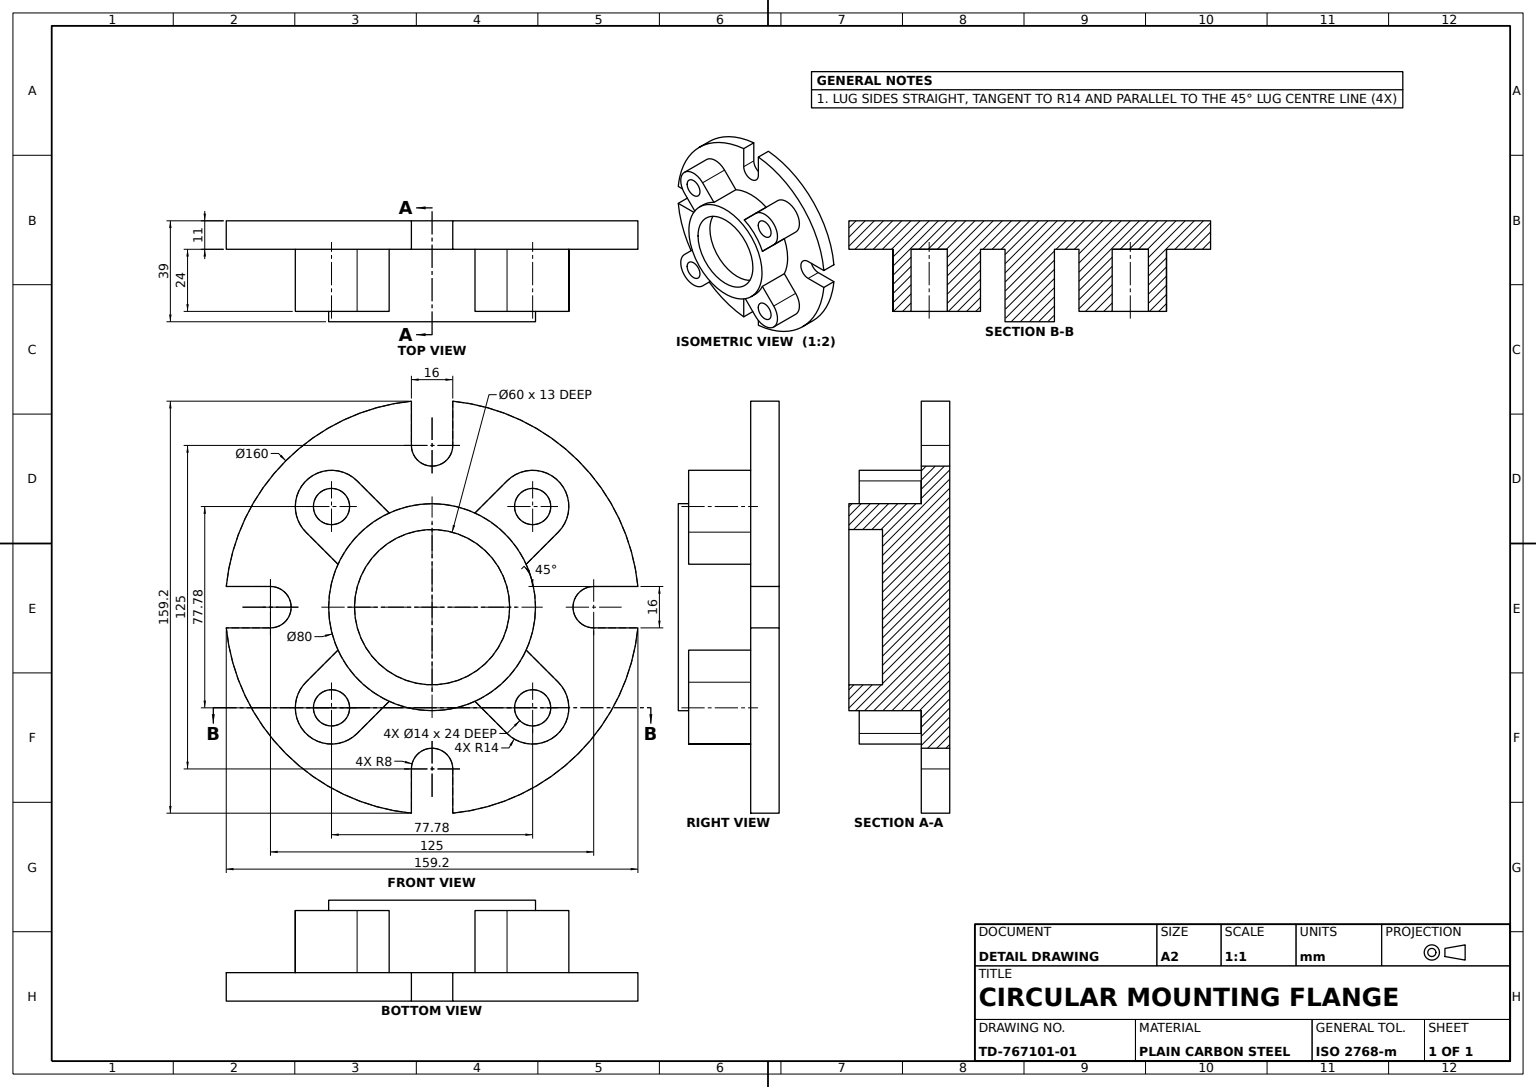
ISO-10303-21;
HEADER;
FILE_DESCRIPTION((''),'2;1');
FILE_NAME('','',(''),(''),'','','');
FILE_SCHEMA(('AUTOMOTIVE_DESIGN'));
ENDSEC;
DATA;
#1=APPLICATION_CONTEXT('');
#2=PRODUCT_CONTEXT('',#1,'mechanical');
#3=PRODUCT('','','',(#2));
#4=PRODUCT_DEFINITION_FORMATION('','',#3);
#5=PRODUCT_DEFINITION_CONTEXT('',#1,'design');
#6=PRODUCT_DEFINITION('','',#4,#5);
#7=PRODUCT_DEFINITION_SHAPE('','',#6);
#8=(LENGTH_UNIT()NAMED_UNIT(*)SI_UNIT(.MILLI.,.METRE.));
#9=(NAMED_UNIT(*)PLANE_ANGLE_UNIT()SI_UNIT($,.RADIAN.));
#10=(NAMED_UNIT(*)SI_UNIT($,.STERADIAN.)SOLID_ANGLE_UNIT());
#11=UNCERTAINTY_MEASURE_WITH_UNIT(LENGTH_MEASURE(1.E-05),#8,'distance_accuracy_value','');
#12=(GEOMETRIC_REPRESENTATION_CONTEXT(3)GLOBAL_UNCERTAINTY_ASSIGNED_CONTEXT((#11))GLOBAL_UNIT_ASSIGNED_CONTEXT((#8,#9,#10))REPRESENTATION_CONTEXT('',''));
#13=CARTESIAN_POINT('',(-79.598995,-8.,0.));
#14=VERTEX_POINT('',#13);
#15=CARTESIAN_POINT('',(-79.598995,-8.,11.));
#16=VERTEX_POINT('',#15);
#17=CARTESIAN_POINT('',(-79.598995,-8.,-13.));
#18=DIRECTION('',(0.,0.,1.));
#19=VECTOR('',#18,1000.);
#20=LINE('',#17,#19);
#21=EDGE_CURVE('',#14,#16,#20,.T.);
#22=ORIENTED_EDGE('',*,*,#21,.F.);
#23=CARTESIAN_POINT('',(-8.,-79.598995,0.));
#24=VERTEX_POINT('',#23);
#25=CARTESIAN_POINT('',(0.,0.,0.));
#26=DIRECTION('',(1.,0.,0.));
#27=AXIS2_PLACEMENT_3D('',#25,#18,#26);
#28=CIRCLE('',#27,80.);
#29=EDGE_CURVE('',#14,#24,#28,.T.);
#30=ORIENTED_EDGE('',*,*,#29,.T.);
#31=CARTESIAN_POINT('',(-8.,-79.598995,11.));
#32=VERTEX_POINT('',#31);
#33=CARTESIAN_POINT('',(-8.,-79.598995,-13.));
#34=LINE('',#33,#19);
#35=EDGE_CURVE('',#24,#32,#34,.T.);
#36=ORIENTED_EDGE('',*,*,#35,.T.);
#37=CARTESIAN_POINT('',(0.,0.,11.));
#38=AXIS2_PLACEMENT_3D('',#37,#18,#26);
#39=CIRCLE('',#38,80.);
#40=EDGE_CURVE('',#16,#32,#39,.T.);
#41=ORIENTED_EDGE('',*,*,#40,.F.);
#42=EDGE_LOOP('',(#22,#30,#36,#41));
#43=FACE_OUTER_BOUND('',#42,.T.);
#44=DIRECTION('',(0.,0.,-1.));
#45=DIRECTION('',(-1.,0.,0.));
#46=AXIS2_PLACEMENT_3D('',#37,#44,#45);
#47=CYLINDRICAL_SURFACE('',#46,80.);
#48=ADVANCED_FACE('',(#43),#47,.T.);
#49=CARTESIAN_POINT('',(-28.991378,-48.790368,35.));
#50=VERTEX_POINT('',#49);
#51=CARTESIAN_POINT('',(-16.595788,-36.394778,35.));
#52=VERTEX_POINT('',#51);
#53=DIRECTION('',(0.707106781,0.707106781,0.));
#54=VECTOR('',#53,1000.);
#55=LINE('',#51,#54);
#56=EDGE_CURVE('',#50,#52,#55,.T.);
#57=ORIENTED_EDGE('',*,*,#56,.F.);
#58=CARTESIAN_POINT('',(-28.991378,-48.790368,11.));
#59=VERTEX_POINT('',#58);
#60=VECTOR('',#44,1000.);
#61=LINE('',#49,#60);
#62=EDGE_CURVE('',#50,#59,#61,.T.);
#63=ORIENTED_EDGE('',*,*,#62,.T.);
#64=CARTESIAN_POINT('',(-16.595788,-36.394778,11.));
#65=VERTEX_POINT('',#64);
#66=LINE('',#64,#54);
#67=EDGE_CURVE('',#59,#65,#66,.T.);
#68=ORIENTED_EDGE('',*,*,#67,.T.);
#69=LINE('',#51,#60);
#70=EDGE_CURVE('',#52,#65,#69,.T.);
#71=ORIENTED_EDGE('',*,*,#70,.F.);
#72=EDGE_LOOP('',(#57,#63,#68,#71));
#73=FACE_OUTER_BOUND('',#72,.T.);
#74=DIRECTION('',(-0.707106781,0.707106781,0.));
#75=DIRECTION('',(-0.707106781,-0.707106781,0.));
#76=AXIS2_PLACEMENT_3D('',#51,#74,#75);
#77=PLANE('',#76);
#78=ADVANCED_FACE('',(#73),#77,.F.);
#79=CARTESIAN_POINT('',(45.890873,-38.890873,35.));
#80=VERTEX_POINT('',#79);
#81=CARTESIAN_POINT('',(31.890873,-38.890873,35.));
#82=VERTEX_POINT('',#81);
#83=CARTESIAN_POINT('',(38.890873,-38.890873,35.));
#84=DIRECTION('',(0.,-1.,0.));
#85=AXIS2_PLACEMENT_3D('',#83,#18,#84);
#86=CIRCLE('',#85,7.);
#87=EDGE_CURVE('',#80,#82,#86,.T.);
#88=ORIENTED_EDGE('',*,*,#87,.F.);
#89=EDGE_CURVE('',#82,#80,#86,.T.);
#90=ORIENTED_EDGE('',*,*,#89,.F.);
#91=EDGE_LOOP('',(#88,#90));
#92=FACE_BOUND('',#91,.T.);
#93=CARTESIAN_POINT('',(36.394778,-16.595788,35.));
#94=VERTEX_POINT('',#93);
#95=CARTESIAN_POINT('',(16.595788,-36.394778,35.));
#96=VERTEX_POINT('',#95);
#97=CARTESIAN_POINT('',(0.,0.,35.));
#98=AXIS2_PLACEMENT_3D('',#97,#44,#84);
#99=CIRCLE('',#98,40.);
#100=EDGE_CURVE('',#94,#96,#99,.T.);
#101=ORIENTED_EDGE('',*,*,#100,.T.);
#102=CARTESIAN_POINT('',(28.991378,-48.790368,35.));
#103=VERTEX_POINT('',#102);
#104=DIRECTION('',(0.707106781,-0.707106781,0.));
#105=VECTOR('',#104,1000.);
#106=LINE('',#95,#105);
#107=EDGE_CURVE('',#96,#103,#106,.T.);
#108=ORIENTED_EDGE('',*,*,#107,.T.);
#109=CARTESIAN_POINT('',(48.790368,-28.991378,35.));
#110=VERTEX_POINT('',#109);
#111=CIRCLE('',#85,14.);
#112=EDGE_CURVE('',#103,#110,#111,.T.);
#113=ORIENTED_EDGE('',*,*,#112,.T.);
#114=VECTOR('',#74,1000.);
#115=LINE('',#93,#114);
#116=EDGE_CURVE('',#110,#94,#115,.T.);
#117=ORIENTED_EDGE('',*,*,#116,.T.);
#118=EDGE_LOOP('',(#101,#108,#113,#117));
#119=FACE_OUTER_BOUND('',#118,.T.);
#120=AXIS2_PLACEMENT_3D('',#97,#18,#84);
#121=PLANE('',#120);
#122=ADVANCED_FACE('',(#92,#119),#121,.T.);
#123=CARTESIAN_POINT('',(62.5,8.,0.));
#124=VERTEX_POINT('',#123);
#125=CARTESIAN_POINT('',(62.5,8.,11.));
#126=VERTEX_POINT('',#125);
#127=CARTESIAN_POINT('',(62.5,8.,-13.));
#128=LINE('',#127,#19);
#129=EDGE_CURVE('',#124,#126,#128,.T.);
#130=ORIENTED_EDGE('',*,*,#129,.T.);
#131=CARTESIAN_POINT('',(62.5,-8.,11.));
#132=VERTEX_POINT('',#131);
#133=CARTESIAN_POINT('',(62.5,0.,11.));
#134=AXIS2_PLACEMENT_3D('',#133,#18,#26);
#135=CIRCLE('',#134,8.);
#136=EDGE_CURVE('',#126,#132,#135,.T.);
#137=ORIENTED_EDGE('',*,*,#136,.T.);
#138=CARTESIAN_POINT('',(62.5,-8.,0.));
#139=VERTEX_POINT('',#138);
#140=CARTESIAN_POINT('',(62.5,-8.,-13.));
#141=LINE('',#140,#19);
#142=EDGE_CURVE('',#139,#132,#141,.T.);
#143=ORIENTED_EDGE('',*,*,#142,.F.);
#144=CARTESIAN_POINT('',(62.5,0.,0.));
#145=AXIS2_PLACEMENT_3D('',#144,#18,#26);
#146=CIRCLE('',#145,8.);
#147=EDGE_CURVE('',#124,#139,#146,.T.);
#148=ORIENTED_EDGE('',*,*,#147,.F.);
#149=EDGE_LOOP('',(#130,#137,#143,#148));
#150=FACE_OUTER_BOUND('',#149,.T.);
#151=CARTESIAN_POINT('',(62.5,0.,-13.));
#152=AXIS2_PLACEMENT_3D('',#151,#18,#26);
#153=CYLINDRICAL_SURFACE('',#152,8.);
#154=ADVANCED_FACE('',(#150),#153,.F.);
#155=CARTESIAN_POINT('',(16.595788,36.394778,35.));
#156=VERTEX_POINT('',#155);
#157=CARTESIAN_POINT('',(36.394778,16.595788,35.));
#158=VERTEX_POINT('',#157);
#159=AXIS2_PLACEMENT_3D('',#97,#44,#26);
#160=CIRCLE('',#159,40.);
#161=EDGE_CURVE('',#156,#158,#160,.T.);
#162=ORIENTED_EDGE('',*,*,#161,.T.);
#163=CARTESIAN_POINT('',(48.790368,28.991378,35.));
#164=VERTEX_POINT('',#163);
#165=LINE('',#157,#54);
#166=EDGE_CURVE('',#158,#164,#165,.T.);
#167=ORIENTED_EDGE('',*,*,#166,.T.);
#168=CARTESIAN_POINT('',(28.991378,48.790368,35.));
#169=VERTEX_POINT('',#168);
#170=CARTESIAN_POINT('',(38.890873,38.890873,35.));
#171=AXIS2_PLACEMENT_3D('',#170,#18,#26);
#172=CIRCLE('',#171,14.);
#173=EDGE_CURVE('',#164,#169,#172,.T.);
#174=ORIENTED_EDGE('',*,*,#173,.T.);
#175=VECTOR('',#75,1000.);
#176=LINE('',#155,#175);
#177=EDGE_CURVE('',#169,#156,#176,.T.);
#178=ORIENTED_EDGE('',*,*,#177,.T.);
#179=EDGE_LOOP('',(#162,#167,#174,#178));
#180=FACE_OUTER_BOUND('',#179,.T.);
#181=CARTESIAN_POINT('',(31.890873,38.890873,35.));
#182=VERTEX_POINT('',#181);
#183=CARTESIAN_POINT('',(45.890873,38.890873,35.));
#184=VERTEX_POINT('',#183);
#185=CIRCLE('',#171,7.);
#186=EDGE_CURVE('',#182,#184,#185,.T.);
#187=ORIENTED_EDGE('',*,*,#186,.F.);
#188=EDGE_CURVE('',#184,#182,#185,.T.);
#189=ORIENTED_EDGE('',*,*,#188,.F.);
#190=EDGE_LOOP('',(#187,#189));
#191=FACE_BOUND('',#190,.T.);
#192=AXIS2_PLACEMENT_3D('',#97,#18,#26);
#193=PLANE('',#192);
#194=ADVANCED_FACE('',(#180,#191),#193,.T.);
#195=ORIENTED_EDGE('',*,*,#166,.F.);
#196=CARTESIAN_POINT('',(36.394778,16.595788,11.));
#197=VERTEX_POINT('',#196);
#198=LINE('',#157,#60);
#199=EDGE_CURVE('',#158,#197,#198,.T.);
#200=ORIENTED_EDGE('',*,*,#199,.T.);
#201=CARTESIAN_POINT('',(48.790368,28.991378,11.));
#202=VERTEX_POINT('',#201);
#203=LINE('',#196,#54);
#204=EDGE_CURVE('',#197,#202,#203,.T.);
#205=ORIENTED_EDGE('',*,*,#204,.T.);
#206=LINE('',#163,#60);
#207=EDGE_CURVE('',#164,#202,#206,.T.);
#208=ORIENTED_EDGE('',*,*,#207,.F.);
#209=EDGE_LOOP('',(#195,#200,#205,#208));
#210=FACE_OUTER_BOUND('',#209,.T.);
#211=AXIS2_PLACEMENT_3D('',#157,#74,#75);
#212=PLANE('',#211);
#213=ADVANCED_FACE('',(#210),#212,.F.);
#214=CARTESIAN_POINT('',(31.890873,-38.890873,11.));
#215=VERTEX_POINT('',#214);
#216=CARTESIAN_POINT('',(45.890873,-38.890873,11.));
#217=VERTEX_POINT('',#216);
#218=CARTESIAN_POINT('',(38.890873,-38.890873,11.));
#219=AXIS2_PLACEMENT_3D('',#218,#44,#26);
#220=CIRCLE('',#219,7.);
#221=EDGE_CURVE('',#215,#217,#220,.T.);
#222=ORIENTED_EDGE('',*,*,#221,.F.);
#223=EDGE_CURVE('',#217,#215,#220,.T.);
#224=ORIENTED_EDGE('',*,*,#223,.F.);
#225=EDGE_LOOP('',(#222,#224));
#226=FACE_OUTER_BOUND('',#225,.T.);
#227=PLANE('',#38);
#228=ADVANCED_FACE('',(#226),#227,.T.);
#229=CARTESIAN_POINT('',(8.,-79.598995,11.));
#230=VERTEX_POINT('',#229);
#231=CARTESIAN_POINT('',(79.598995,-8.,11.));
#232=VERTEX_POINT('',#231);
#233=EDGE_CURVE('',#230,#232,#39,.T.);
#234=ORIENTED_EDGE('',*,*,#233,.F.);
#235=CARTESIAN_POINT('',(8.,-79.598995,0.));
#236=VERTEX_POINT('',#235);
#237=CARTESIAN_POINT('',(8.,-79.598995,-13.));
#238=LINE('',#237,#19);
#239=EDGE_CURVE('',#236,#230,#238,.T.);
#240=ORIENTED_EDGE('',*,*,#239,.F.);
#241=CARTESIAN_POINT('',(79.598995,-8.,0.));
#242=VERTEX_POINT('',#241);
#243=EDGE_CURVE('',#236,#242,#28,.T.);
#244=ORIENTED_EDGE('',*,*,#243,.T.);
#245=CARTESIAN_POINT('',(79.598995,-8.,-13.));
#246=LINE('',#245,#19);
#247=EDGE_CURVE('',#242,#232,#246,.T.);
#248=ORIENTED_EDGE('',*,*,#247,.T.);
#249=EDGE_LOOP('',(#234,#240,#244,#248));
#250=FACE_OUTER_BOUND('',#249,.T.);
#251=ADVANCED_FACE('',(#250),#47,.T.);
#252=CARTESIAN_POINT('',(-45.890873,-38.890873,35.));
#253=VERTEX_POINT('',#252);
#254=CARTESIAN_POINT('',(-45.890873,-38.890873,11.));
#255=VERTEX_POINT('',#254);
#256=LINE('',#252,#60);
#257=EDGE_CURVE('',#253,#255,#256,.T.);
#258=ORIENTED_EDGE('',*,*,#257,.T.);
#259=CARTESIAN_POINT('',(-31.890873,-38.890873,11.));
#260=VERTEX_POINT('',#259);
#261=CARTESIAN_POINT('',(-38.890873,-38.890873,11.));
#262=AXIS2_PLACEMENT_3D('',#261,#44,#26);
#263=CIRCLE('',#262,7.);
#264=EDGE_CURVE('',#255,#260,#263,.T.);
#265=ORIENTED_EDGE('',*,*,#264,.T.);
#266=CARTESIAN_POINT('',(-31.890873,-38.890873,35.));
#267=VERTEX_POINT('',#266);
#268=LINE('',#266,#60);
#269=EDGE_CURVE('',#267,#260,#268,.T.);
#270=ORIENTED_EDGE('',*,*,#269,.F.);
#271=CARTESIAN_POINT('',(-38.890873,-38.890873,35.));
#272=AXIS2_PLACEMENT_3D('',#271,#18,#45);
#273=CIRCLE('',#272,7.);
#274=EDGE_CURVE('',#267,#253,#273,.T.);
#275=ORIENTED_EDGE('',*,*,#274,.T.);
#276=EDGE_LOOP('',(#258,#265,#270,#275));
#277=FACE_OUTER_BOUND('',#276,.T.);
#278=AXIS2_PLACEMENT_3D('',#271,#44,#45);
#279=CYLINDRICAL_SURFACE('',#278,7.);
#280=ADVANCED_FACE('',(#277),#279,.F.);
#281=CARTESIAN_POINT('',(-45.890873,38.890873,11.));
#282=VERTEX_POINT('',#281);
#283=CARTESIAN_POINT('',(-31.890873,38.890873,11.));
#284=VERTEX_POINT('',#283);
#285=CARTESIAN_POINT('',(-38.890873,38.890873,11.));
#286=AXIS2_PLACEMENT_3D('',#285,#44,#26);
#287=CIRCLE('',#286,7.);
#288=EDGE_CURVE('',#282,#284,#287,.T.);
#289=ORIENTED_EDGE('',*,*,#288,.T.);
#290=CARTESIAN_POINT('',(-31.890873,38.890873,35.));
#291=VERTEX_POINT('',#290);
#292=LINE('',#290,#60);
#293=EDGE_CURVE('',#291,#284,#292,.T.);
#294=ORIENTED_EDGE('',*,*,#293,.F.);
#295=CARTESIAN_POINT('',(-45.890873,38.890873,35.));
#296=VERTEX_POINT('',#295);
#297=CARTESIAN_POINT('',(-38.890873,38.890873,35.));
#298=DIRECTION('',(0.,1.,0.));
#299=AXIS2_PLACEMENT_3D('',#297,#18,#298);
#300=CIRCLE('',#299,7.);
#301=EDGE_CURVE('',#291,#296,#300,.T.);
#302=ORIENTED_EDGE('',*,*,#301,.T.);
#303=LINE('',#295,#60);
#304=EDGE_CURVE('',#296,#282,#303,.T.);
#305=ORIENTED_EDGE('',*,*,#304,.T.);
#306=EDGE_LOOP('',(#289,#294,#302,#305));
#307=FACE_OUTER_BOUND('',#306,.T.);
#308=AXIS2_PLACEMENT_3D('',#297,#44,#45);
#309=CYLINDRICAL_SURFACE('',#308,7.);
#310=ADVANCED_FACE('',(#307),#309,.F.);
#311=ORIENTED_EDGE('',*,*,#87,.T.);
#312=LINE('',#81,#60);
#313=EDGE_CURVE('',#82,#215,#312,.T.);
#314=ORIENTED_EDGE('',*,*,#313,.T.);
#315=ORIENTED_EDGE('',*,*,#221,.T.);
#316=LINE('',#79,#60);
#317=EDGE_CURVE('',#80,#217,#316,.T.);
#318=ORIENTED_EDGE('',*,*,#317,.F.);
#319=EDGE_LOOP('',(#311,#314,#315,#318));
#320=FACE_OUTER_BOUND('',#319,.T.);
#321=AXIS2_PLACEMENT_3D('',#83,#44,#45);
#322=CYLINDRICAL_SURFACE('',#321,7.);
#323=ADVANCED_FACE('',(#320),#322,.F.);
#324=CARTESIAN_POINT('',(-28.991378,48.790368,35.));
#325=VERTEX_POINT('',#324);
#326=CARTESIAN_POINT('',(-52.890873,38.890873,35.));
#327=VERTEX_POINT('',#326);
#328=CIRCLE('',#299,14.);
#329=EDGE_CURVE('',#325,#327,#328,.T.);
#330=ORIENTED_EDGE('',*,*,#329,.F.);
#331=CARTESIAN_POINT('',(-28.991378,48.790368,11.));
#332=VERTEX_POINT('',#331);
#333=LINE('',#324,#60);
#334=EDGE_CURVE('',#325,#332,#333,.T.);
#335=ORIENTED_EDGE('',*,*,#334,.T.);
#336=CARTESIAN_POINT('',(-52.890873,38.890873,11.));
#337=VERTEX_POINT('',#336);
#338=AXIS2_PLACEMENT_3D('',#285,#18,#298);
#339=CIRCLE('',#338,14.);
#340=EDGE_CURVE('',#332,#337,#339,.T.);
#341=ORIENTED_EDGE('',*,*,#340,.T.);
#342=LINE('',#326,#60);
#343=EDGE_CURVE('',#327,#337,#342,.T.);
#344=ORIENTED_EDGE('',*,*,#343,.F.);
#345=EDGE_LOOP('',(#330,#335,#341,#344));
#346=FACE_OUTER_BOUND('',#345,.T.);
#347=CYLINDRICAL_SURFACE('',#308,14.);
#348=ADVANCED_FACE('',(#346),#347,.T.);
#349=CARTESIAN_POINT('',(0.,-8.,0.));
#350=VECTOR('',#26,1000.);
#351=LINE('',#349,#350);
#352=EDGE_CURVE('',#139,#242,#351,.T.);
#353=ORIENTED_EDGE('',*,*,#352,.T.);
#354=ORIENTED_EDGE('',*,*,#243,.F.);
#355=CARTESIAN_POINT('',(8.,-62.5,0.));
#356=VERTEX_POINT('',#355);
#357=CARTESIAN_POINT('',(8.,0.,0.));
#358=VECTOR('',#298,1000.);
#359=LINE('',#357,#358);
#360=EDGE_CURVE('',#236,#356,#359,.T.);
#361=ORIENTED_EDGE('',*,*,#360,.T.);
#362=CARTESIAN_POINT('',(-8.,-62.5,0.));
#363=VERTEX_POINT('',#362);
#364=CARTESIAN_POINT('',(0.,-62.5,0.));
#365=AXIS2_PLACEMENT_3D('',#364,#18,#26);
#366=CIRCLE('',#365,8.);
#367=EDGE_CURVE('',#356,#363,#366,.T.);
#368=ORIENTED_EDGE('',*,*,#367,.T.);
#369=CARTESIAN_POINT('',(-8.,0.,0.));
#370=VECTOR('',#84,1000.);
#371=LINE('',#369,#370);
#372=EDGE_CURVE('',#363,#24,#371,.T.);
#373=ORIENTED_EDGE('',*,*,#372,.T.);
#374=ORIENTED_EDGE('',*,*,#29,.F.);
#375=CARTESIAN_POINT('',(-62.5,-8.,0.));
#376=VERTEX_POINT('',#375);
#377=EDGE_CURVE('',#14,#376,#351,.T.);
#378=ORIENTED_EDGE('',*,*,#377,.T.);
#379=CARTESIAN_POINT('',(-54.5,0.,0.));
#380=VERTEX_POINT('',#379);
#381=CARTESIAN_POINT('',(-62.5,0.,0.));
#382=AXIS2_PLACEMENT_3D('',#381,#18,#26);
#383=CIRCLE('',#382,8.);
#384=EDGE_CURVE('',#376,#380,#383,.T.);
#385=ORIENTED_EDGE('',*,*,#384,.T.);
#386=CARTESIAN_POINT('',(-62.5,8.,0.));
#387=VERTEX_POINT('',#386);
#388=EDGE_CURVE('',#380,#387,#383,.T.);
#389=ORIENTED_EDGE('',*,*,#388,.T.);
#390=CARTESIAN_POINT('',(-79.598995,8.,0.));
#391=VERTEX_POINT('',#390);
#392=CARTESIAN_POINT('',(0.,8.,0.));
#393=VECTOR('',#45,1000.);
#394=LINE('',#392,#393);
#395=EDGE_CURVE('',#387,#391,#394,.T.);
#396=ORIENTED_EDGE('',*,*,#395,.T.);
#397=CARTESIAN_POINT('',(-8.,79.598995,0.));
#398=VERTEX_POINT('',#397);
#399=EDGE_CURVE('',#398,#391,#28,.T.);
#400=ORIENTED_EDGE('',*,*,#399,.F.);
#401=CARTESIAN_POINT('',(-8.,62.5,0.));
#402=VERTEX_POINT('',#401);
#403=EDGE_CURVE('',#398,#402,#371,.T.);
#404=ORIENTED_EDGE('',*,*,#403,.T.);
#405=CARTESIAN_POINT('',(8.,62.5,0.));
#406=VERTEX_POINT('',#405);
#407=CARTESIAN_POINT('',(0.,62.5,0.));
#408=AXIS2_PLACEMENT_3D('',#407,#18,#26);
#409=CIRCLE('',#408,8.);
#410=EDGE_CURVE('',#402,#406,#409,.T.);
#411=ORIENTED_EDGE('',*,*,#410,.T.);
#412=CARTESIAN_POINT('',(8.,79.598995,0.));
#413=VERTEX_POINT('',#412);
#414=EDGE_CURVE('',#406,#413,#359,.T.);
#415=ORIENTED_EDGE('',*,*,#414,.T.);
#416=CARTESIAN_POINT('',(79.598995,8.,0.));
#417=VERTEX_POINT('',#416);
#418=EDGE_CURVE('',#417,#413,#28,.T.);
#419=ORIENTED_EDGE('',*,*,#418,.F.);
#420=EDGE_CURVE('',#417,#124,#394,.T.);
#421=ORIENTED_EDGE('',*,*,#420,.T.);
#422=ORIENTED_EDGE('',*,*,#147,.T.);
#423=EDGE_LOOP('',(#353,#354,#361,#368,#373,#374,#378,#385,#389,#396,#400,#404,#411,#415,#419,#421,#422));
#424=FACE_OUTER_BOUND('',#423,.T.);
#425=PLANE('',#27);
#426=ADVANCED_FACE('',(#424),#425,.F.);
#427=CARTESIAN_POINT('',(-48.790368,28.991378,35.));
#428=VERTEX_POINT('',#427);
#429=CARTESIAN_POINT('',(-48.790368,28.991378,11.));
#430=VERTEX_POINT('',#429);
#431=LINE('',#427,#60);
#432=EDGE_CURVE('',#428,#430,#431,.T.);
#433=ORIENTED_EDGE('',*,*,#432,.T.);
#434=CARTESIAN_POINT('',(-36.394778,16.595788,11.));
#435=VERTEX_POINT('',#434);
#436=LINE('',#434,#105);
#437=EDGE_CURVE('',#430,#435,#436,.T.);
#438=ORIENTED_EDGE('',*,*,#437,.T.);
#439=CARTESIAN_POINT('',(-36.394778,16.595788,35.));
#440=VERTEX_POINT('',#439);
#441=LINE('',#439,#60);
#442=EDGE_CURVE('',#440,#435,#441,.T.);
#443=ORIENTED_EDGE('',*,*,#442,.F.);
#444=LINE('',#439,#105);
#445=EDGE_CURVE('',#428,#440,#444,.T.);
#446=ORIENTED_EDGE('',*,*,#445,.F.);
#447=EDGE_LOOP('',(#433,#438,#443,#446));
#448=FACE_OUTER_BOUND('',#447,.T.);
#449=AXIS2_PLACEMENT_3D('',#439,#53,#74);
#450=PLANE('',#449);
#451=ADVANCED_FACE('',(#448),#450,.F.);
#452=CARTESIAN_POINT('',(-8.,-62.5,11.));
#453=VERTEX_POINT('',#452);
#454=CARTESIAN_POINT('',(-8.,-62.5,-13.));
#455=LINE('',#454,#19);
#456=EDGE_CURVE('',#363,#453,#455,.T.);
#457=ORIENTED_EDGE('',*,*,#456,.T.);
#458=LINE('',#452,#370);
#459=EDGE_CURVE('',#453,#32,#458,.T.);
#460=ORIENTED_EDGE('',*,*,#459,.T.);
#461=ORIENTED_EDGE('',*,*,#35,.F.);
#462=ORIENTED_EDGE('',*,*,#372,.F.);
#463=EDGE_LOOP('',(#457,#460,#461,#462));
#464=FACE_OUTER_BOUND('',#463,.T.);
#465=AXIS2_PLACEMENT_3D('',#454,#45,#84);
#466=PLANE('',#465);
#467=ADVANCED_FACE('',(#464),#466,.F.);
#468=CARTESIAN_POINT('',(-8.,79.598995,11.));
#469=VERTEX_POINT('',#468);
#470=CARTESIAN_POINT('',(-79.598995,8.,11.));
#471=VERTEX_POINT('',#470);
#472=EDGE_CURVE('',#469,#471,#39,.T.);
#473=ORIENTED_EDGE('',*,*,#472,.F.);
#474=CARTESIAN_POINT('',(-8.,79.598995,-13.));
#475=LINE('',#474,#19);
#476=EDGE_CURVE('',#398,#469,#475,.T.);
#477=ORIENTED_EDGE('',*,*,#476,.F.);
#478=ORIENTED_EDGE('',*,*,#399,.T.);
#479=CARTESIAN_POINT('',(-79.598995,8.,-13.));
#480=LINE('',#479,#19);
#481=EDGE_CURVE('',#391,#471,#480,.T.);
#482=ORIENTED_EDGE('',*,*,#481,.T.);
#483=EDGE_LOOP('',(#473,#477,#478,#482));
#484=FACE_OUTER_BOUND('',#483,.T.);
#485=ADVANCED_FACE('',(#484),#47,.T.);
#486=CARTESIAN_POINT('',(-62.5,8.,11.));
#487=VERTEX_POINT('',#486);
#488=CARTESIAN_POINT('',(-62.5,8.,-13.));
#489=LINE('',#488,#19);
#490=EDGE_CURVE('',#387,#487,#489,.T.);
#491=ORIENTED_EDGE('',*,*,#490,.F.);
#492=ORIENTED_EDGE('',*,*,#388,.F.);
#493=CARTESIAN_POINT('',(-54.5,0.,11.));
#494=VERTEX_POINT('',#493);
#495=CARTESIAN_POINT('',(-54.5,0.,-13.));
#496=LINE('',#495,#19);
#497=EDGE_CURVE('',#380,#494,#496,.T.);
#498=ORIENTED_EDGE('',*,*,#497,.T.);
#499=CARTESIAN_POINT('',(-62.5,0.,11.));
#500=AXIS2_PLACEMENT_3D('',#499,#18,#45);
#501=CIRCLE('',#500,8.);
#502=EDGE_CURVE('',#494,#487,#501,.T.);
#503=ORIENTED_EDGE('',*,*,#502,.T.);
#504=EDGE_LOOP('',(#491,#492,#498,#503));
#505=FACE_OUTER_BOUND('',#504,.T.);
#506=CARTESIAN_POINT('',(-62.5,0.,-13.));
#507=AXIS2_PLACEMENT_3D('',#506,#18,#26);
#508=CYLINDRICAL_SURFACE('',#507,8.);
#509=ADVANCED_FACE('',(#505),#508,.F.);
#510=ORIENTED_EDGE('',*,*,#161,.F.);
#511=CARTESIAN_POINT('',(16.595788,36.394778,11.));
#512=VERTEX_POINT('',#511);
#513=LINE('',#155,#60);
#514=EDGE_CURVE('',#156,#512,#513,.T.);
#515=ORIENTED_EDGE('',*,*,#514,.T.);
#516=CARTESIAN_POINT('',(-16.595788,36.394778,11.));
#517=VERTEX_POINT('',#516);
#518=CIRCLE('',#38,40.);
#519=EDGE_CURVE('',#512,#517,#518,.T.);
#520=ORIENTED_EDGE('',*,*,#519,.T.);
#521=CARTESIAN_POINT('',(-16.595788,36.394778,35.));
#522=VERTEX_POINT('',#521);
#523=LINE('',#521,#60);
#524=EDGE_CURVE('',#522,#517,#523,.T.);
#525=ORIENTED_EDGE('',*,*,#524,.F.);
#526=AXIS2_PLACEMENT_3D('',#97,#44,#298);
#527=CIRCLE('',#526,40.);
#528=EDGE_CURVE('',#440,#522,#527,.T.);
#529=ORIENTED_EDGE('',*,*,#528,.F.);
#530=ORIENTED_EDGE('',*,*,#442,.T.);
#531=CARTESIAN_POINT('',(-40.,0.,11.));
#532=VERTEX_POINT('',#531);
#533=EDGE_CURVE('',#435,#532,#518,.T.);
#534=ORIENTED_EDGE('',*,*,#533,.T.);
#535=CARTESIAN_POINT('',(-40.,0.,39.));
#536=VERTEX_POINT('',#535);
#537=LINE('',#535,#60);
#538=EDGE_CURVE('',#536,#532,#537,.T.);
#539=ORIENTED_EDGE('',*,*,#538,.F.);
#540=CARTESIAN_POINT('',(40.,0.,39.));
#541=VERTEX_POINT('',#540);
#542=CARTESIAN_POINT('',(0.,0.,39.));
#543=AXIS2_PLACEMENT_3D('',#542,#18,#26);
#544=CIRCLE('',#543,40.);
#545=EDGE_CURVE('',#541,#536,#544,.T.);
#546=ORIENTED_EDGE('',*,*,#545,.F.);
#547=CARTESIAN_POINT('',(40.,0.,11.));
#548=VERTEX_POINT('',#547);
#549=LINE('',#540,#60);
#550=EDGE_CURVE('',#541,#548,#549,.T.);
#551=ORIENTED_EDGE('',*,*,#550,.T.);
#552=EDGE_CURVE('',#548,#197,#518,.T.);
#553=ORIENTED_EDGE('',*,*,#552,.T.);
#554=ORIENTED_EDGE('',*,*,#199,.F.);
#555=EDGE_LOOP('',(#510,#515,#520,#525,#529,#530,#534,#539,#546,#551,#553,#554));
#556=FACE_OUTER_BOUND('',#555,.T.);
#557=AXIS2_PLACEMENT_3D('',#542,#44,#45);
#558=CYLINDRICAL_SURFACE('',#557,40.);
#559=ADVANCED_FACE('',(#556),#558,.T.);
#560=CARTESIAN_POINT('',(79.598995,8.,11.));
#561=VERTEX_POINT('',#560);
#562=LINE('',#125,#393);
#563=EDGE_CURVE('',#561,#126,#562,.T.);
#564=ORIENTED_EDGE('',*,*,#563,.F.);
#565=CARTESIAN_POINT('',(8.,79.598995,11.));
#566=VERTEX_POINT('',#565);
#567=EDGE_CURVE('',#561,#566,#39,.T.);
#568=ORIENTED_EDGE('',*,*,#567,.T.);
#569=CARTESIAN_POINT('',(8.,62.5,11.));
#570=VERTEX_POINT('',#569);
#571=LINE('',#569,#358);
#572=EDGE_CURVE('',#570,#566,#571,.T.);
#573=ORIENTED_EDGE('',*,*,#572,.F.);
#574=CARTESIAN_POINT('',(-8.,62.5,11.));
#575=VERTEX_POINT('',#574);
#576=CARTESIAN_POINT('',(0.,62.5,11.));
#577=AXIS2_PLACEMENT_3D('',#576,#18,#298);
#578=CIRCLE('',#577,8.);
#579=EDGE_CURVE('',#575,#570,#578,.T.);
#580=ORIENTED_EDGE('',*,*,#579,.F.);
#581=LINE('',#574,#370);
#582=EDGE_CURVE('',#469,#575,#581,.T.);
#583=ORIENTED_EDGE('',*,*,#582,.F.);
#584=ORIENTED_EDGE('',*,*,#472,.T.);
#585=LINE('',#486,#393);
#586=EDGE_CURVE('',#487,#471,#585,.T.);
#587=ORIENTED_EDGE('',*,*,#586,.F.);
#588=ORIENTED_EDGE('',*,*,#502,.F.);
#589=CARTESIAN_POINT('',(-62.5,-8.,11.));
#590=VERTEX_POINT('',#589);
#591=EDGE_CURVE('',#590,#494,#501,.T.);
#592=ORIENTED_EDGE('',*,*,#591,.F.);
#593=LINE('',#589,#350);
#594=EDGE_CURVE('',#16,#590,#593,.T.);
#595=ORIENTED_EDGE('',*,*,#594,.F.);
#596=ORIENTED_EDGE('',*,*,#40,.T.);
#597=ORIENTED_EDGE('',*,*,#459,.F.);
#598=CARTESIAN_POINT('',(8.,-62.5,11.));
#599=VERTEX_POINT('',#598);
#600=CARTESIAN_POINT('',(0.,-62.5,11.));
#601=AXIS2_PLACEMENT_3D('',#600,#18,#84);
#602=CIRCLE('',#601,8.);
#603=EDGE_CURVE('',#599,#453,#602,.T.);
#604=ORIENTED_EDGE('',*,*,#603,.F.);
#605=LINE('',#598,#358);
#606=EDGE_CURVE('',#230,#599,#605,.T.);
#607=ORIENTED_EDGE('',*,*,#606,.F.);
#608=ORIENTED_EDGE('',*,*,#233,.T.);
#609=LINE('',#131,#350);
#610=EDGE_CURVE('',#132,#232,#609,.T.);
#611=ORIENTED_EDGE('',*,*,#610,.F.);
#612=ORIENTED_EDGE('',*,*,#136,.F.);
#613=EDGE_LOOP('',(#564,#568,#573,#580,#583,#584,#587,#588,#592,#595,#596,#597,#604,#607,#608,#611,#612));
#614=FACE_OUTER_BOUND('',#613,.T.);
#615=CARTESIAN_POINT('',(-52.890873,-38.890873,11.));
#616=VERTEX_POINT('',#615);
#617=AXIS2_PLACEMENT_3D('',#261,#18,#45);
#618=CIRCLE('',#617,14.);
#619=EDGE_CURVE('',#616,#59,#618,.T.);
#620=ORIENTED_EDGE('',*,*,#619,.F.);
#621=CARTESIAN_POINT('',(-48.790368,-28.991378,11.));
#622=VERTEX_POINT('',#621);
#623=EDGE_CURVE('',#622,#616,#618,.T.);
#624=ORIENTED_EDGE('',*,*,#623,.F.);
#625=CARTESIAN_POINT('',(-36.394778,-16.595788,11.));
#626=VERTEX_POINT('',#625);
#627=LINE('',#625,#175);
#628=EDGE_CURVE('',#626,#622,#627,.T.);
#629=ORIENTED_EDGE('',*,*,#628,.F.);
#630=EDGE_CURVE('',#532,#626,#518,.T.);
#631=ORIENTED_EDGE('',*,*,#630,.F.);
#632=ORIENTED_EDGE('',*,*,#533,.F.);
#633=ORIENTED_EDGE('',*,*,#437,.F.);
#634=EDGE_CURVE('',#337,#430,#339,.T.);
#635=ORIENTED_EDGE('',*,*,#634,.F.);
#636=ORIENTED_EDGE('',*,*,#340,.F.);
#637=LINE('',#516,#114);
#638=EDGE_CURVE('',#517,#332,#637,.T.);
#639=ORIENTED_EDGE('',*,*,#638,.F.);
#640=ORIENTED_EDGE('',*,*,#519,.F.);
#641=CARTESIAN_POINT('',(28.991378,48.790368,11.));
#642=VERTEX_POINT('',#641);
#643=LINE('',#511,#175);
#644=EDGE_CURVE('',#642,#512,#643,.T.);
#645=ORIENTED_EDGE('',*,*,#644,.F.);
#646=CARTESIAN_POINT('',(38.890873,38.890873,11.));
#647=AXIS2_PLACEMENT_3D('',#646,#18,#26);
#648=CIRCLE('',#647,14.);
#649=EDGE_CURVE('',#202,#642,#648,.T.);
#650=ORIENTED_EDGE('',*,*,#649,.F.);
#651=ORIENTED_EDGE('',*,*,#204,.F.);
#652=ORIENTED_EDGE('',*,*,#552,.F.);
#653=CARTESIAN_POINT('',(36.394778,-16.595788,11.));
#654=VERTEX_POINT('',#653);
#655=EDGE_CURVE('',#654,#548,#518,.T.);
#656=ORIENTED_EDGE('',*,*,#655,.F.);
#657=CARTESIAN_POINT('',(48.790368,-28.991378,11.));
#658=VERTEX_POINT('',#657);
#659=LINE('',#653,#114);
#660=EDGE_CURVE('',#658,#654,#659,.T.);
#661=ORIENTED_EDGE('',*,*,#660,.F.);
#662=CARTESIAN_POINT('',(28.991378,-48.790368,11.));
#663=VERTEX_POINT('',#662);
#664=AXIS2_PLACEMENT_3D('',#218,#18,#84);
#665=CIRCLE('',#664,14.);
#666=EDGE_CURVE('',#663,#658,#665,.T.);
#667=ORIENTED_EDGE('',*,*,#666,.F.);
#668=CARTESIAN_POINT('',(16.595788,-36.394778,11.));
#669=VERTEX_POINT('',#668);
#670=LINE('',#668,#105);
#671=EDGE_CURVE('',#669,#663,#670,.T.);
#672=ORIENTED_EDGE('',*,*,#671,.F.);
#673=EDGE_CURVE('',#65,#669,#518,.T.);
#674=ORIENTED_EDGE('',*,*,#673,.F.);
#675=ORIENTED_EDGE('',*,*,#67,.F.);
#676=EDGE_LOOP('',(#620,#624,#629,#631,#632,#633,#635,#636,#639,#640,#645,#650,#651,#652,#656,#661,#667,#672,#674,#675));
#677=FACE_BOUND('',#676,.T.);
#678=ADVANCED_FACE('',(#614,#677),#227,.T.);
#679=CARTESIAN_POINT('',(30.,0.,39.));
#680=VERTEX_POINT('',#679);
#681=CARTESIAN_POINT('',(30.,0.,26.));
#682=VERTEX_POINT('',#681);
#683=LINE('',#679,#60);
#684=EDGE_CURVE('',#680,#682,#683,.T.);
#685=ORIENTED_EDGE('',*,*,#684,.T.);
#686=CARTESIAN_POINT('',(-30.,0.,26.));
#687=VERTEX_POINT('',#686);
#688=CARTESIAN_POINT('',(0.,0.,26.));
#689=AXIS2_PLACEMENT_3D('',#688,#18,#26);
#690=CIRCLE('',#689,30.);
#691=EDGE_CURVE('',#687,#682,#690,.T.);
#692=ORIENTED_EDGE('',*,*,#691,.F.);
#693=CARTESIAN_POINT('',(-30.,0.,39.));
#694=VERTEX_POINT('',#693);
#695=LINE('',#693,#60);
#696=EDGE_CURVE('',#694,#687,#695,.T.);
#697=ORIENTED_EDGE('',*,*,#696,.F.);
#698=CIRCLE('',#543,30.);
#699=EDGE_CURVE('',#694,#680,#698,.T.);
#700=ORIENTED_EDGE('',*,*,#699,.T.);
#701=EDGE_LOOP('',(#685,#692,#697,#700));
#702=FACE_OUTER_BOUND('',#701,.T.);
#703=CYLINDRICAL_SURFACE('',#557,30.);
#704=ADVANCED_FACE('',(#702),#703,.F.);
#705=CARTESIAN_POINT('',(8.,79.598995,-13.));
#706=LINE('',#705,#19);
#707=EDGE_CURVE('',#413,#566,#706,.T.);
#708=ORIENTED_EDGE('',*,*,#707,.T.);
#709=ORIENTED_EDGE('',*,*,#567,.F.);
#710=CARTESIAN_POINT('',(79.598995,8.,-13.));
#711=LINE('',#710,#19);
#712=EDGE_CURVE('',#417,#561,#711,.T.);
#713=ORIENTED_EDGE('',*,*,#712,.F.);
#714=ORIENTED_EDGE('',*,*,#418,.T.);
#715=EDGE_LOOP('',(#708,#709,#713,#714));
#716=FACE_OUTER_BOUND('',#715,.T.);
#717=ADVANCED_FACE('',(#716),#47,.T.);
#718=CARTESIAN_POINT('',(-48.790368,-28.991378,35.));
#719=VERTEX_POINT('',#718);
#720=LINE('',#718,#60);
#721=EDGE_CURVE('',#719,#622,#720,.T.);
#722=ORIENTED_EDGE('',*,*,#721,.F.);
#723=CARTESIAN_POINT('',(-36.394778,-16.595788,35.));
#724=VERTEX_POINT('',#723);
#725=LINE('',#723,#175);
#726=EDGE_CURVE('',#724,#719,#725,.T.);
#727=ORIENTED_EDGE('',*,*,#726,.F.);
#728=LINE('',#723,#60);
#729=EDGE_CURVE('',#724,#626,#728,.T.);
#730=ORIENTED_EDGE('',*,*,#729,.T.);
#731=ORIENTED_EDGE('',*,*,#628,.T.);
#732=EDGE_LOOP('',(#722,#727,#730,#731));
#733=FACE_OUTER_BOUND('',#732,.T.);
#734=AXIS2_PLACEMENT_3D('',#723,#104,#53);
#735=PLANE('',#734);
#736=ADVANCED_FACE('',(#733),#735,.F.);
#737=ORIENTED_EDGE('',*,*,#606,.T.);
#738=CARTESIAN_POINT('',(8.,-62.5,-13.));
#739=LINE('',#738,#19);
#740=EDGE_CURVE('',#356,#599,#739,.T.);
#741=ORIENTED_EDGE('',*,*,#740,.F.);
#742=ORIENTED_EDGE('',*,*,#360,.F.);
#743=ORIENTED_EDGE('',*,*,#239,.T.);
#744=EDGE_LOOP('',(#737,#741,#742,#743));
#745=FACE_OUTER_BOUND('',#744,.T.);
#746=AXIS2_PLACEMENT_3D('',#738,#26,#298);
#747=PLANE('',#746);
#748=ADVANCED_FACE('',(#745),#747,.F.);
#749=ORIENTED_EDGE('',*,*,#173,.F.);
#750=ORIENTED_EDGE('',*,*,#207,.T.);
#751=ORIENTED_EDGE('',*,*,#649,.T.);
#752=LINE('',#168,#60);
#753=EDGE_CURVE('',#169,#642,#752,.T.);
#754=ORIENTED_EDGE('',*,*,#753,.F.);
#755=EDGE_LOOP('',(#749,#750,#751,#754));
#756=FACE_OUTER_BOUND('',#755,.T.);
#757=AXIS2_PLACEMENT_3D('',#170,#44,#45);
#758=CYLINDRICAL_SURFACE('',#757,14.);
#759=ADVANCED_FACE('',(#756),#758,.T.);
#760=EDGE_CURVE('',#296,#291,#300,.T.);
#761=ORIENTED_EDGE('',*,*,#760,.T.);
#762=ORIENTED_EDGE('',*,*,#293,.T.);
#763=EDGE_CURVE('',#284,#282,#287,.T.);
#764=ORIENTED_EDGE('',*,*,#763,.T.);
#765=ORIENTED_EDGE('',*,*,#304,.F.);
#766=EDGE_LOOP('',(#761,#762,#764,#765));
#767=FACE_OUTER_BOUND('',#766,.T.);
#768=ADVANCED_FACE('',(#767),#309,.F.);
#769=ORIENTED_EDGE('',*,*,#186,.T.);
#770=CARTESIAN_POINT('',(45.890873,38.890873,11.));
#771=VERTEX_POINT('',#770);
#772=LINE('',#183,#60);
#773=EDGE_CURVE('',#184,#771,#772,.T.);
#774=ORIENTED_EDGE('',*,*,#773,.T.);
#775=CARTESIAN_POINT('',(31.890873,38.890873,11.));
#776=VERTEX_POINT('',#775);
#777=AXIS2_PLACEMENT_3D('',#646,#44,#26);
#778=CIRCLE('',#777,7.);
#779=EDGE_CURVE('',#771,#776,#778,.T.);
#780=ORIENTED_EDGE('',*,*,#779,.T.);
#781=LINE('',#181,#60);
#782=EDGE_CURVE('',#182,#776,#781,.T.);
#783=ORIENTED_EDGE('',*,*,#782,.F.);
#784=EDGE_LOOP('',(#769,#774,#780,#783));
#785=FACE_OUTER_BOUND('',#784,.T.);
#786=CYLINDRICAL_SURFACE('',#757,7.);
#787=ADVANCED_FACE('',(#785),#786,.F.);
#788=ORIENTED_EDGE('',*,*,#514,.F.);
#789=ORIENTED_EDGE('',*,*,#177,.F.);
#790=ORIENTED_EDGE('',*,*,#753,.T.);
#791=ORIENTED_EDGE('',*,*,#644,.T.);
#792=EDGE_LOOP('',(#788,#789,#790,#791));
#793=FACE_OUTER_BOUND('',#792,.T.);
#794=AXIS2_PLACEMENT_3D('',#155,#104,#53);
#795=PLANE('',#794);
#796=ADVANCED_FACE('',(#793),#795,.F.);
#797=EDGE_CURVE('',#253,#267,#273,.T.);
#798=ORIENTED_EDGE('',*,*,#797,.T.);
#799=ORIENTED_EDGE('',*,*,#269,.T.);
#800=EDGE_CURVE('',#260,#255,#263,.T.);
#801=ORIENTED_EDGE('',*,*,#800,.T.);
#802=ORIENTED_EDGE('',*,*,#257,.F.);
#803=EDGE_LOOP('',(#798,#799,#801,#802));
#804=FACE_OUTER_BOUND('',#803,.T.);
#805=ADVANCED_FACE('',(#804),#279,.F.);
#806=ORIENTED_EDGE('',*,*,#696,.T.);
#807=EDGE_CURVE('',#682,#687,#690,.T.);
#808=ORIENTED_EDGE('',*,*,#807,.F.);
#809=ORIENTED_EDGE('',*,*,#684,.F.);
#810=EDGE_CURVE('',#680,#694,#698,.T.);
#811=ORIENTED_EDGE('',*,*,#810,.T.);
#812=EDGE_LOOP('',(#806,#808,#809,#811));
#813=FACE_OUTER_BOUND('',#812,.T.);
#814=ADVANCED_FACE('',(#813),#703,.F.);
#815=ORIENTED_EDGE('',*,*,#367,.F.);
#816=ORIENTED_EDGE('',*,*,#740,.T.);
#817=ORIENTED_EDGE('',*,*,#603,.T.);
#818=ORIENTED_EDGE('',*,*,#456,.F.);
#819=EDGE_LOOP('',(#815,#816,#817,#818));
#820=FACE_OUTER_BOUND('',#819,.T.);
#821=CARTESIAN_POINT('',(0.,-62.5,-13.));
#822=AXIS2_PLACEMENT_3D('',#821,#18,#26);
#823=CYLINDRICAL_SURFACE('',#822,8.);
#824=ADVANCED_FACE('',(#820),#823,.F.);
#825=ORIENTED_EDGE('',*,*,#334,.F.);
#826=LINE('',#521,#114);
#827=EDGE_CURVE('',#522,#325,#826,.T.);
#828=ORIENTED_EDGE('',*,*,#827,.F.);
#829=ORIENTED_EDGE('',*,*,#524,.T.);
#830=ORIENTED_EDGE('',*,*,#638,.T.);
#831=EDGE_LOOP('',(#825,#828,#829,#830));
#832=FACE_OUTER_BOUND('',#831,.T.);
#833=AXIS2_PLACEMENT_3D('',#521,#75,#104);
#834=PLANE('',#833);
#835=ADVANCED_FACE('',(#832),#834,.F.);
#836=ORIENTED_EDGE('',*,*,#288,.F.);
#837=ORIENTED_EDGE('',*,*,#763,.F.);
#838=EDGE_LOOP('',(#836,#837));
#839=FACE_OUTER_BOUND('',#838,.T.);
#840=ADVANCED_FACE('',(#839),#227,.T.);
#841=EDGE_CURVE('',#327,#428,#328,.T.);
#842=ORIENTED_EDGE('',*,*,#841,.T.);
#843=ORIENTED_EDGE('',*,*,#445,.T.);
#844=ORIENTED_EDGE('',*,*,#528,.T.);
#845=ORIENTED_EDGE('',*,*,#827,.T.);
#846=ORIENTED_EDGE('',*,*,#329,.T.);
#847=EDGE_LOOP('',(#842,#843,#844,#845,#846));
#848=FACE_OUTER_BOUND('',#847,.T.);
#849=ORIENTED_EDGE('',*,*,#301,.F.);
#850=ORIENTED_EDGE('',*,*,#760,.F.);
#851=EDGE_LOOP('',(#849,#850));
#852=FACE_BOUND('',#851,.T.);
#853=AXIS2_PLACEMENT_3D('',#97,#18,#298);
#854=PLANE('',#853);
#855=ADVANCED_FACE('',(#848,#852),#854,.T.);
#856=ORIENTED_EDGE('',*,*,#420,.F.);
#857=ORIENTED_EDGE('',*,*,#712,.T.);
#858=ORIENTED_EDGE('',*,*,#563,.T.);
#859=ORIENTED_EDGE('',*,*,#129,.F.);
#860=EDGE_LOOP('',(#856,#857,#858,#859));
#861=FACE_OUTER_BOUND('',#860,.T.);
#862=AXIS2_PLACEMENT_3D('',#127,#298,#18);
#863=PLANE('',#862);
#864=ADVANCED_FACE('',(#861),#863,.F.);
#865=ORIENTED_EDGE('',*,*,#691,.T.);
#866=ORIENTED_EDGE('',*,*,#807,.T.);
#867=EDGE_LOOP('',(#865,#866));
#868=FACE_OUTER_BOUND('',#867,.T.);
#869=PLANE('',#689);
#870=ADVANCED_FACE('',(#868),#869,.T.);
#871=ORIENTED_EDGE('',*,*,#142,.T.);
#872=ORIENTED_EDGE('',*,*,#610,.T.);
#873=ORIENTED_EDGE('',*,*,#247,.F.);
#874=ORIENTED_EDGE('',*,*,#352,.F.);
#875=EDGE_LOOP('',(#871,#872,#873,#874));
#876=FACE_OUTER_BOUND('',#875,.T.);
#877=AXIS2_PLACEMENT_3D('',#140,#84,#44);
#878=PLANE('',#877);
#879=ADVANCED_FACE('',(#876),#878,.F.);
#880=ORIENTED_EDGE('',*,*,#432,.F.);
#881=ORIENTED_EDGE('',*,*,#841,.F.);
#882=ORIENTED_EDGE('',*,*,#343,.T.);
#883=ORIENTED_EDGE('',*,*,#634,.T.);
#884=EDGE_LOOP('',(#880,#881,#882,#883));
#885=FACE_OUTER_BOUND('',#884,.T.);
#886=ADVANCED_FACE('',(#885),#347,.T.);
#887=ORIENTED_EDGE('',*,*,#810,.F.);
#888=ORIENTED_EDGE('',*,*,#699,.F.);
#889=EDGE_LOOP('',(#887,#888));
#890=FACE_BOUND('',#889,.T.);
#891=ORIENTED_EDGE('',*,*,#545,.T.);
#892=EDGE_CURVE('',#536,#541,#544,.T.);
#893=ORIENTED_EDGE('',*,*,#892,.T.);
#894=EDGE_LOOP('',(#891,#893));
#895=FACE_OUTER_BOUND('',#894,.T.);
#896=PLANE('',#543);
#897=ADVANCED_FACE('',(#890,#895),#896,.T.);
#898=ORIENTED_EDGE('',*,*,#623,.T.);
#899=CARTESIAN_POINT('',(-52.890873,-38.890873,35.));
#900=VERTEX_POINT('',#899);
#901=LINE('',#899,#60);
#902=EDGE_CURVE('',#900,#616,#901,.T.);
#903=ORIENTED_EDGE('',*,*,#902,.F.);
#904=CIRCLE('',#272,14.);
#905=EDGE_CURVE('',#719,#900,#904,.T.);
#906=ORIENTED_EDGE('',*,*,#905,.F.);
#907=ORIENTED_EDGE('',*,*,#721,.T.);
#908=EDGE_LOOP('',(#898,#903,#906,#907));
#909=FACE_OUTER_BOUND('',#908,.T.);
#910=CYLINDRICAL_SURFACE('',#278,14.);
#911=ADVANCED_FACE('',(#909),#910,.T.);
#912=ORIENTED_EDGE('',*,*,#497,.F.);
#913=ORIENTED_EDGE('',*,*,#384,.F.);
#914=CARTESIAN_POINT('',(-62.5,-8.,-13.));
#915=LINE('',#914,#19);
#916=EDGE_CURVE('',#376,#590,#915,.T.);
#917=ORIENTED_EDGE('',*,*,#916,.T.);
#918=ORIENTED_EDGE('',*,*,#591,.T.);
#919=EDGE_LOOP('',(#912,#913,#917,#918));
#920=FACE_OUTER_BOUND('',#919,.T.);
#921=ADVANCED_FACE('',(#920),#508,.F.);
#922=ORIENTED_EDGE('',*,*,#619,.T.);
#923=ORIENTED_EDGE('',*,*,#62,.F.);
#924=EDGE_CURVE('',#900,#50,#904,.T.);
#925=ORIENTED_EDGE('',*,*,#924,.F.);
#926=ORIENTED_EDGE('',*,*,#902,.T.);
#927=EDGE_LOOP('',(#922,#923,#925,#926));
#928=FACE_OUTER_BOUND('',#927,.T.);
#929=ADVANCED_FACE('',(#928),#910,.T.);
#930=ORIENTED_EDGE('',*,*,#671,.T.);
#931=LINE('',#102,#60);
#932=EDGE_CURVE('',#103,#663,#931,.T.);
#933=ORIENTED_EDGE('',*,*,#932,.F.);
#934=ORIENTED_EDGE('',*,*,#107,.F.);
#935=LINE('',#95,#60);
#936=EDGE_CURVE('',#96,#669,#935,.T.);
#937=ORIENTED_EDGE('',*,*,#936,.T.);
#938=EDGE_LOOP('',(#930,#933,#934,#937));
#939=FACE_OUTER_BOUND('',#938,.T.);
#940=AXIS2_PLACEMENT_3D('',#95,#53,#74);
#941=PLANE('',#940);
#942=ADVANCED_FACE('',(#939),#941,.F.);
#943=ORIENTED_EDGE('',*,*,#264,.F.);
#944=ORIENTED_EDGE('',*,*,#800,.F.);
#945=EDGE_LOOP('',(#943,#944));
#946=FACE_OUTER_BOUND('',#945,.T.);
#947=ADVANCED_FACE('',(#946),#227,.T.);
#948=ORIENTED_EDGE('',*,*,#782,.T.);
#949=EDGE_CURVE('',#776,#771,#778,.T.);
#950=ORIENTED_EDGE('',*,*,#949,.T.);
#951=ORIENTED_EDGE('',*,*,#773,.F.);
#952=ORIENTED_EDGE('',*,*,#188,.T.);
#953=EDGE_LOOP('',(#948,#950,#951,#952));
#954=FACE_OUTER_BOUND('',#953,.T.);
#955=ADVANCED_FACE('',(#954),#786,.F.);
#956=CARTESIAN_POINT('',(-8.,62.5,-13.));
#957=LINE('',#956,#19);
#958=EDGE_CURVE('',#402,#575,#957,.T.);
#959=ORIENTED_EDGE('',*,*,#958,.F.);
#960=ORIENTED_EDGE('',*,*,#403,.F.);
#961=ORIENTED_EDGE('',*,*,#476,.T.);
#962=ORIENTED_EDGE('',*,*,#582,.T.);
#963=EDGE_LOOP('',(#959,#960,#961,#962));
#964=FACE_OUTER_BOUND('',#963,.T.);
#965=AXIS2_PLACEMENT_3D('',#956,#45,#84);
#966=PLANE('',#965);
#967=ADVANCED_FACE('',(#964),#966,.F.);
#968=ORIENTED_EDGE('',*,*,#797,.F.);
#969=ORIENTED_EDGE('',*,*,#274,.F.);
#970=EDGE_LOOP('',(#968,#969));
#971=FACE_BOUND('',#970,.T.);
#972=ORIENTED_EDGE('',*,*,#56,.T.);
#973=AXIS2_PLACEMENT_3D('',#97,#44,#45);
#974=CIRCLE('',#973,40.);
#975=EDGE_CURVE('',#52,#724,#974,.T.);
#976=ORIENTED_EDGE('',*,*,#975,.T.);
#977=ORIENTED_EDGE('',*,*,#726,.T.);
#978=ORIENTED_EDGE('',*,*,#905,.T.);
#979=ORIENTED_EDGE('',*,*,#924,.T.);
#980=EDGE_LOOP('',(#972,#976,#977,#978,#979));
#981=FACE_OUTER_BOUND('',#980,.T.);
#982=AXIS2_PLACEMENT_3D('',#97,#18,#45);
#983=PLANE('',#982);
#984=ADVANCED_FACE('',(#971,#981),#983,.T.);
#985=ORIENTED_EDGE('',*,*,#21,.T.);
#986=ORIENTED_EDGE('',*,*,#594,.T.);
#987=ORIENTED_EDGE('',*,*,#916,.F.);
#988=ORIENTED_EDGE('',*,*,#377,.F.);
#989=EDGE_LOOP('',(#985,#986,#987,#988));
#990=FACE_OUTER_BOUND('',#989,.T.);
#991=AXIS2_PLACEMENT_3D('',#914,#84,#44);
#992=PLANE('',#991);
#993=ADVANCED_FACE('',(#990),#992,.F.);
#994=ORIENTED_EDGE('',*,*,#673,.T.);
#995=ORIENTED_EDGE('',*,*,#936,.F.);
#996=ORIENTED_EDGE('',*,*,#100,.F.);
#997=LINE('',#93,#60);
#998=EDGE_CURVE('',#94,#654,#997,.T.);
#999=ORIENTED_EDGE('',*,*,#998,.T.);
#1000=ORIENTED_EDGE('',*,*,#655,.T.);
#1001=ORIENTED_EDGE('',*,*,#550,.F.);
#1002=ORIENTED_EDGE('',*,*,#892,.F.);
#1003=ORIENTED_EDGE('',*,*,#538,.T.);
#1004=ORIENTED_EDGE('',*,*,#630,.T.);
#1005=ORIENTED_EDGE('',*,*,#729,.F.);
#1006=ORIENTED_EDGE('',*,*,#975,.F.);
#1007=ORIENTED_EDGE('',*,*,#70,.T.);
#1008=EDGE_LOOP('',(#994,#995,#996,#999,#1000,#1001,#1002,#1003,#1004,#1005,#1006,#1007));
#1009=FACE_OUTER_BOUND('',#1008,.T.);
#1010=ADVANCED_FACE('',(#1009),#558,.T.);
#1011=ORIENTED_EDGE('',*,*,#958,.T.);
#1012=ORIENTED_EDGE('',*,*,#579,.T.);
#1013=CARTESIAN_POINT('',(8.,62.5,-13.));
#1014=LINE('',#1013,#19);
#1015=EDGE_CURVE('',#406,#570,#1014,.T.);
#1016=ORIENTED_EDGE('',*,*,#1015,.F.);
#1017=ORIENTED_EDGE('',*,*,#410,.F.);
#1018=EDGE_LOOP('',(#1011,#1012,#1016,#1017));
#1019=FACE_OUTER_BOUND('',#1018,.T.);
#1020=CARTESIAN_POINT('',(0.,62.5,-13.));
#1021=AXIS2_PLACEMENT_3D('',#1020,#18,#26);
#1022=CYLINDRICAL_SURFACE('',#1021,8.);
#1023=ADVANCED_FACE('',(#1019),#1022,.F.);
#1024=ORIENTED_EDGE('',*,*,#660,.T.);
#1025=ORIENTED_EDGE('',*,*,#998,.F.);
#1026=ORIENTED_EDGE('',*,*,#116,.F.);
#1027=LINE('',#109,#60);
#1028=EDGE_CURVE('',#110,#658,#1027,.T.);
#1029=ORIENTED_EDGE('',*,*,#1028,.T.);
#1030=EDGE_LOOP('',(#1024,#1025,#1026,#1029));
#1031=FACE_OUTER_BOUND('',#1030,.T.);
#1032=AXIS2_PLACEMENT_3D('',#93,#75,#104);
#1033=PLANE('',#1032);
#1034=ADVANCED_FACE('',(#1031),#1033,.F.);
#1035=ORIENTED_EDGE('',*,*,#490,.T.);
#1036=ORIENTED_EDGE('',*,*,#586,.T.);
#1037=ORIENTED_EDGE('',*,*,#481,.F.);
#1038=ORIENTED_EDGE('',*,*,#395,.F.);
#1039=EDGE_LOOP('',(#1035,#1036,#1037,#1038));
#1040=FACE_OUTER_BOUND('',#1039,.T.);
#1041=AXIS2_PLACEMENT_3D('',#488,#298,#18);
#1042=PLANE('',#1041);
#1043=ADVANCED_FACE('',(#1040),#1042,.F.);
#1044=ORIENTED_EDGE('',*,*,#932,.T.);
#1045=ORIENTED_EDGE('',*,*,#666,.T.);
#1046=ORIENTED_EDGE('',*,*,#1028,.F.);
#1047=ORIENTED_EDGE('',*,*,#112,.F.);
#1048=EDGE_LOOP('',(#1044,#1045,#1046,#1047));
#1049=FACE_OUTER_BOUND('',#1048,.T.);
#1050=CYLINDRICAL_SURFACE('',#321,14.);
#1051=ADVANCED_FACE('',(#1049),#1050,.T.);
#1052=ORIENTED_EDGE('',*,*,#779,.F.);
#1053=ORIENTED_EDGE('',*,*,#949,.F.);
#1054=EDGE_LOOP('',(#1052,#1053));
#1055=FACE_OUTER_BOUND('',#1054,.T.);
#1056=ADVANCED_FACE('',(#1055),#227,.T.);
#1057=ORIENTED_EDGE('',*,*,#1015,.T.);
#1058=ORIENTED_EDGE('',*,*,#572,.T.);
#1059=ORIENTED_EDGE('',*,*,#707,.F.);
#1060=ORIENTED_EDGE('',*,*,#414,.F.);
#1061=EDGE_LOOP('',(#1057,#1058,#1059,#1060));
#1062=FACE_OUTER_BOUND('',#1061,.T.);
#1063=AXIS2_PLACEMENT_3D('',#1013,#26,#298);
#1064=PLANE('',#1063);
#1065=ADVANCED_FACE('',(#1062),#1064,.F.);
#1066=ORIENTED_EDGE('',*,*,#317,.T.);
#1067=ORIENTED_EDGE('',*,*,#223,.T.);
#1068=ORIENTED_EDGE('',*,*,#313,.F.);
#1069=ORIENTED_EDGE('',*,*,#89,.T.);
#1070=EDGE_LOOP('',(#1066,#1067,#1068,#1069));
#1071=FACE_OUTER_BOUND('',#1070,.T.);
#1072=ADVANCED_FACE('',(#1071),#322,.F.);
#1073=CLOSED_SHELL('',(#48,#78,#122,#154,#194,#213,#228,#251,#280,#310,#323,#348,#426,#451,#467,#485,#509,#559,#678,#704,#717,#736,#748,#759,#768,#787,#796,#805,#814,#824,#835,#840,#855,#864,#870,#879,#886,#897,#911,#921,#929,#942,#947,#955,#967,#984,#993,#1010,#1023,#1034,#1043,#1051,#1056,#1065,#1072));
#1074=MANIFOLD_SOLID_BREP('',#1073);
#1075=ADVANCED_BREP_SHAPE_REPRESENTATION('',(#1074),#12);
#1076=SHAPE_DEFINITION_REPRESENTATION(#7,#1075);
ENDSEC;
END-ISO-10303-21;
